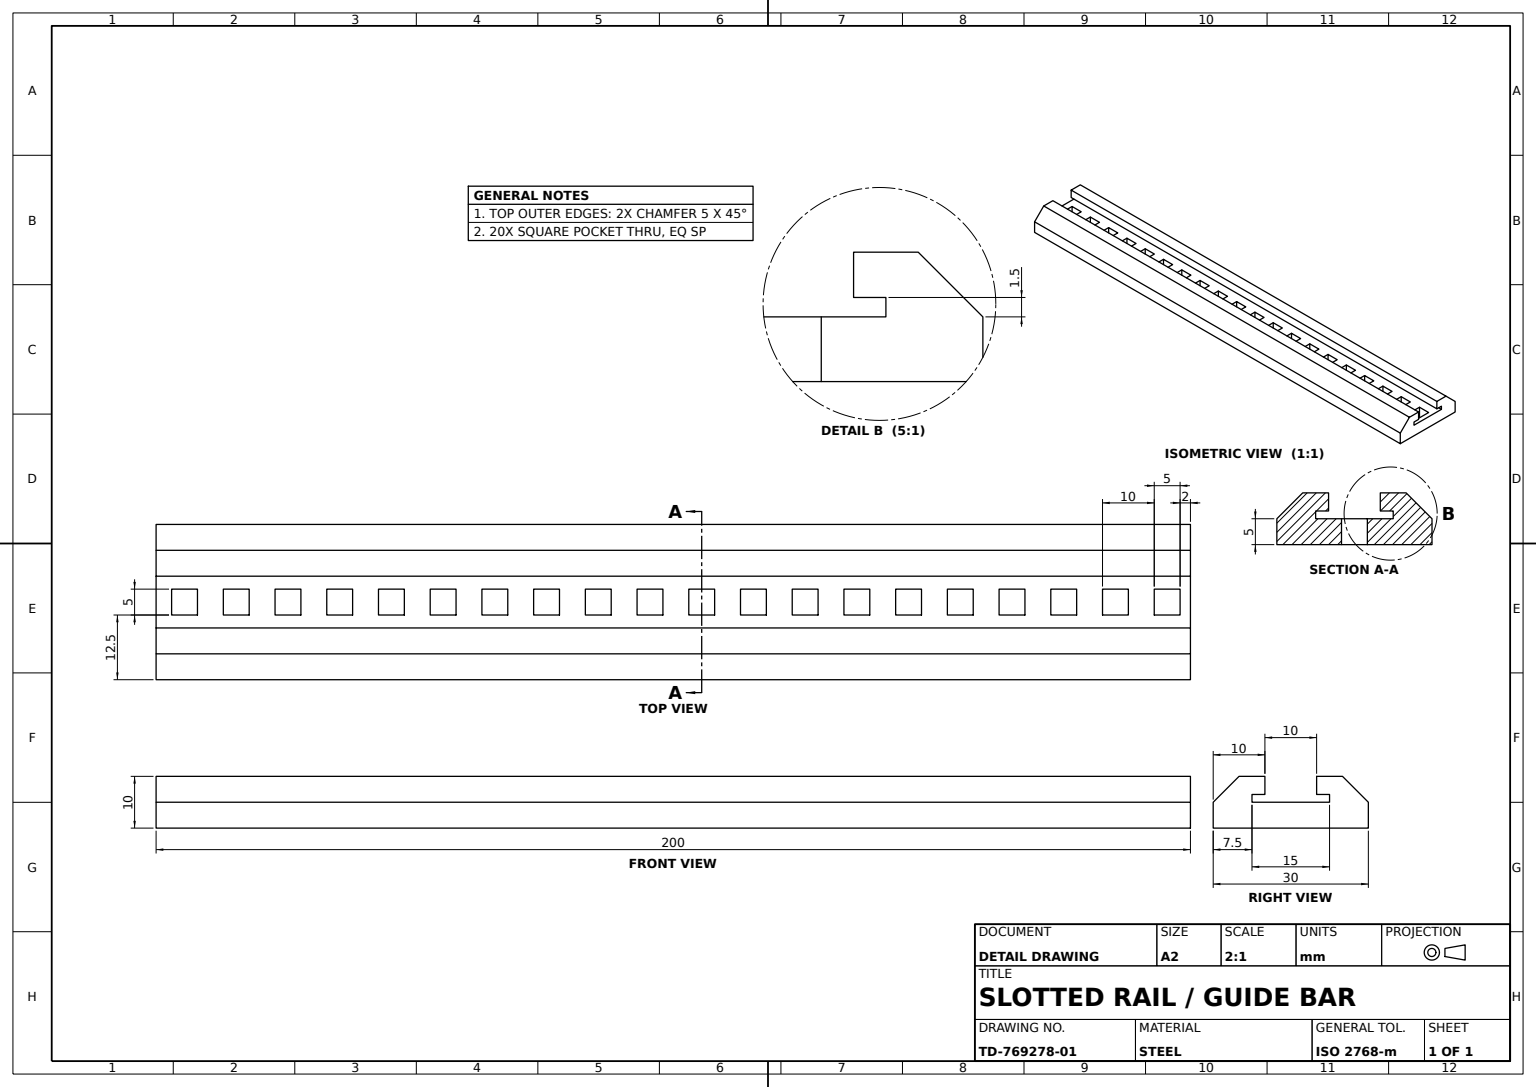
solid
v1 (2.5,-5,47)
v2 (2.5,0,47)
e1 v1 v2 LINE
v3 (2.5,0,42)
e2 v2 v3 LINE
v4 (2.5,-5,42)
e3 v4 v3 LINE
e4 v4 v1 LINE
face PLANE(AX(P(2.5,-5.001,42),D(1,0,0),D(0,0,-1))) rev [e1 e2 -e3 e4]
v5 (-2.5,-5,97)
v6 (-2.5,-5,92)
e5 v5 v6 LINE
v7 (-2.5,0,92)
e6 v6 v7 LINE
v8 (-2.5,0,97)
e7 v7 v8 LINE
e8 v5 v8 LINE
face PLANE(AX(P(-2.5,-5.001,92),D(-1,0,0),D(0,0,1))) rev [e5 e6 e7 -e8]
v9 (2.5,0,-48)
v10 (-2.5,0,-48)
e9 v9 v10 LINE
v11 (-2.5,-5,-48)
e10 v11 v10 LINE
v12 (2.5,-5,-48)
e11 v11 v12 LINE
e12 v12 v9 LINE
face PLANE(AX(P(-2.5,-5.001,-48),D(0,0,-1),D(-1,0,0))) rev [e9 -e10 e11 e12]
v13 (2.5,0,97)
v14 (2.5,0,92)
e13 v13 v14 LINE
v15 (2.5,-5,92)
e14 v15 v14 LINE
v16 (2.5,-5,97)
e15 v15 v16 LINE
e16 v16 v13 LINE
face PLANE(AX(P(2.5,-5.001,92),D(1,0,0),D(0,0,-1))) rev [e13 -e14 e15 e16]
v17 (-2.5,-5,32)
v18 (-2.5,0,32)
e17 v17 v18 LINE
v19 (2.5,-5,32)
e18 v17 v19 LINE
v20 (2.5,0,32)
e19 v19 v20 LINE
e20 v20 v18 LINE
face PLANE(AX(P(-2.5,-5.001,32),D(0,0,-1),D(-1,0,0))) rev [-e17 e18 e19 e20]
v21 (5,1.5,-100)
v22 (5,5,-100)
e21 v21 v22 LINE
v23 (5,1.5,100)
e22 v23 v21 LINE
v24 (5,5,100)
e23 v23 v24 LINE
e24 v24 v22 LINE
face PLANE(AX(P(5,0,-100),D(1,0,0),D(0,0,-1))) rev [-e21 -e22 e23 e24]
v25 (-2.5,-5,2)
v26 (-2.5,0,2)
e25 v25 v26 LINE
v27 (-2.5,0,7)
e26 v26 v27 LINE
v28 (-2.5,-5,7)
e27 v28 v27 LINE
e28 v28 v25 LINE
face PLANE(AX(P(-2.5,-5.001,2),D(-1,0,0),D(0,0,1))) rev [e25 e26 -e27 e28]
v29 (-5,1.5,100)
v30 (-7.5,1.5,100)
e29 v29 v30 LINE
v31 (-7.5,1.5,-100)
e30 v31 v30 LINE
v32 (-5,1.5,-100)
e31 v31 v32 LINE
e32 v32 v29 LINE
face PLANE(AX(P(-7.5,1.5,-100.001),D(0,1,0),D(0,0,1))) rev [e29 -e30 e31 e32]
v33 (-7.5,0,100)
e33 v30 v33 LINE
v34 (-7.5,0,-100)
e34 v34 v33 LINE
e35 v34 v31 LINE
face PLANE(AX(P(-7.5,1.5,-100.001),D(-1,0,0),D(0,0,1))) rev [e33 -e34 e35 e30]
v35 (-2.5,0,-33)
v36 (2.5,0,-33)
e36 v35 v36 LINE
v37 (2.5,-5,-33)
e37 v37 v36 LINE
v38 (-2.5,-5,-33)
e38 v37 v38 LINE
e39 v38 v35 LINE
face PLANE(AX(P(-2.5,-5.001,-33),D(0,0,1),D(1,0,0))) rev [e36 -e37 e38 e39]
v39 (-2.5,-5,-8)
v40 (-2.5,0,-8)
e40 v39 v40 LINE
v41 (-2.5,0,-3)
e41 v40 v41 LINE
v42 (-2.5,-5,-3)
e42 v42 v41 LINE
e43 v42 v39 LINE
face PLANE(AX(P(-2.5,-5.001,-8),D(-1,0,0),D(0,0,1))) rev [e40 e41 -e42 e43]
v43 (2.5,-5,-43)
e44 v12 v43 LINE
v44 (2.5,0,-43)
e45 v43 v44 LINE
e46 v44 v9 LINE
face PLANE(AX(P(2.5,-5.001,-48),D(1,0,0),D(0,0,-1))) rev [-e12 e44 e45 e46]
v45 (-2.5,-5,-28)
v46 (-2.5,0,-28)
e47 v45 v46 LINE
v47 (-2.5,0,-23)
e48 v46 v47 LINE
v48 (-2.5,-5,-23)
e49 v48 v47 LINE
e50 v48 v45 LINE
face PLANE(AX(P(-2.5,-5.001,-28),D(-1,0,0),D(0,0,1))) rev [e47 e48 -e49 e50]
v49 (-2.5,-5,87)
v50 (-2.5,0,87)
e51 v49 v50 LINE
v51 (-2.5,-5,82)
e52 v49 v51 LINE
v52 (-2.5,0,82)
e53 v51 v52 LINE
e54 v52 v50 LINE
face PLANE(AX(P(-2.5,-5.001,82),D(-1,0,0),D(0,0,1))) rev [-e51 e52 e53 e54]
v53 (-2.5,-5,-58)
v54 (-2.5,0,-58)
e55 v53 v54 LINE
v55 (-2.5,0,-53)
e56 v54 v55 LINE
v56 (-2.5,-5,-53)
e57 v56 v55 LINE
e58 v56 v53 LINE
face PLANE(AX(P(-2.5,-5.001,-58),D(-1,0,0),D(0,0,1))) rev [e55 e56 -e57 e58]
v57 (2.5,0,-83)
v58 (2.5,0,-88)
e59 v57 v58 LINE
v59 (2.5,-5,-88)
e60 v59 v58 LINE
v60 (2.5,-5,-83)
e61 v59 v60 LINE
e62 v60 v57 LINE
face PLANE(AX(P(2.5,-5.001,-88),D(1,0,0),D(0,0,-1))) rev [e59 -e60 e61 e62]
v61 (2.5,-5,2)
v62 (2.5,-5,7)
e63 v61 v62 LINE
v63 (2.5,0,7)
e64 v62 v63 LINE
v64 (2.5,0,2)
e65 v63 v64 LINE
e66 v61 v64 LINE
face PLANE(AX(P(2.5,-5.001,2),D(1,0,0),D(0,0,-1))) rev [e63 e64 e65 -e66]
v65 (-2.5,0,-43)
e67 v10 v65 LINE
v66 (-2.5,-5,-43)
e68 v66 v65 LINE
e69 v66 v11 LINE
face PLANE(AX(P(-2.5,-5.001,-48),D(-1,0,0),D(0,0,1))) rev [e10 e67 -e68 e69]
v67 (2.5,0,12)
v68 (-2.5,0,12)
e70 v67 v68 LINE
v69 (-2.5,-5,12)
e71 v69 v68 LINE
v70 (2.5,-5,12)
e72 v69 v70 LINE
e73 v70 v67 LINE
face PLANE(AX(P(-2.5,-5.001,12),D(0,0,-1),D(-1,0,0))) rev [e70 -e71 e72 e73]
v71 (2.5,0,67)
v72 (2.5,0,62)
e74 v71 v72 LINE
v73 (2.5,-5,62)
e75 v73 v72 LINE
v74 (2.5,-5,67)
e76 v73 v74 LINE
e77 v74 v71 LINE
face PLANE(AX(P(2.5,-5.001,62),D(1,0,0),D(0,0,-1))) rev [e74 -e75 e76 e77]
v75 (7.5,1.5,-100)
e78 v21 v75 LINE
v76 (7.5,1.5,100)
e79 v75 v76 LINE
e80 v76 v23 LINE
face PLANE(AX(P(-7.5,1.5,-100.001),D(0,1,0),D(0,0,1))) rev [e78 e79 e80 e22]
e81 v8 v13 LINE
e82 v16 v5 LINE
face PLANE(AX(P(-2.5,-5.001,97),D(0,0,1),D(1,0,0))) rev [e8 e81 -e16 e82]
v77 (2.5,0,-23)
v78 (2.5,0,-28)
e83 v77 v78 LINE
v79 (2.5,-5,-28)
e84 v79 v78 LINE
v80 (2.5,-5,-23)
e85 v79 v80 LINE
e86 v80 v77 LINE
face PLANE(AX(P(2.5,-5.001,-28),D(1,0,0),D(0,0,-1))) rev [e83 -e84 e85 e86]
v81 (-2.5,0,-68)
v82 (-2.5,0,-63)
e87 v81 v82 LINE
v83 (-2.5,-5,-63)
e88 v83 v82 LINE
v84 (-2.5,-5,-68)
e89 v83 v84 LINE
e90 v84 v81 LINE
face PLANE(AX(P(-2.5,-5.001,-68),D(-1,0,0),D(0,0,1))) rev [e87 -e88 e89 e90]
v85 (2.5,-5,22)
v86 (2.5,0,22)
e91 v85 v86 LINE
v87 (2.5,-5,27)
e92 v85 v87 LINE
v88 (2.5,0,27)
e93 v87 v88 LINE
e94 v88 v86 LINE
face PLANE(AX(P(2.5,-5.001,22),D(1,0,0),D(0,0,-1))) rev [-e91 e92 e93 e94]
v89 (2.5,-5,-93)
v90 (2.5,0,-93)
e95 v89 v90 LINE
v91 (2.5,0,-98)
e96 v90 v91 LINE
v92 (2.5,-5,-98)
e97 v92 v91 LINE
e98 v92 v89 LINE
face PLANE(AX(P(2.5,-5.001,-98),D(1,0,0),D(0,0,-1))) rev [e95 e96 -e97 e98]
v93 (2.5,-5,77)
v94 (-2.5,-5,77)
e99 v93 v94 LINE
v95 (-2.5,0,77)
e100 v94 v95 LINE
v96 (2.5,0,77)
e101 v95 v96 LINE
e102 v93 v96 LINE
face PLANE(AX(P(-2.5,-5.001,77),D(0,0,1),D(1,0,0))) rev [e99 e100 e101 -e102]
v97 (2.5,-5,-53)
v98 (2.5,0,-53)
e103 v97 v98 LINE
v99 (2.5,0,-58)
e104 v98 v99 LINE
v100 (2.5,-5,-58)
e105 v100 v99 LINE
e106 v100 v97 LINE
face PLANE(AX(P(2.5,-5.001,-58),D(1,0,0),D(0,0,-1))) rev [e103 e104 -e105 e106]
v101 (-2.5,0,37)
v102 (2.5,0,37)
e107 v101 v102 LINE
v103 (2.5,-5,37)
e108 v103 v102 LINE
v104 (-2.5,-5,37)
e109 v103 v104 LINE
e110 v104 v101 LINE
face PLANE(AX(P(-2.5,-5.001,37),D(0,0,1),D(1,0,0))) rev [e107 -e108 e109 e110]
v105 (-2.5,-5,-93)
v106 (-2.5,-5,-98)
e111 v105 v106 LINE
v107 (-2.5,0,-98)
e112 v106 v107 LINE
v108 (-2.5,0,-93)
e113 v107 v108 LINE
e114 v105 v108 LINE
face PLANE(AX(P(-2.5,-5.001,-98),D(-1,0,0),D(0,0,1))) rev [e111 e112 e113 -e114]
v109 (2.5,-5,52)
v110 (2.5,0,52)
e115 v109 v110 LINE
v111 (-2.5,0,52)
e116 v110 v111 LINE
v112 (-2.5,-5,52)
e117 v112 v111 LINE
e118 v112 v109 LINE
face PLANE(AX(P(-2.5,-5.001,52),D(0,0,-1),D(-1,0,0))) rev [e115 e116 -e117 e118]
e119 v62 v28 LINE
e120 v27 v63 LINE
face PLANE(AX(P(-2.5,-5.001,7),D(0,0,1),D(1,0,0))) rev [e119 e27 e120 -e64]
v113 (2.5,-5,-68)
v114 (2.5,0,-68)
e121 v113 v114 LINE
v115 (2.5,-5,-63)
e122 v113 v115 LINE
v116 (2.5,0,-63)
e123 v115 v116 LINE
e124 v116 v114 LINE
face PLANE(AX(P(2.5,-5.001,-68),D(1,0,0),D(0,0,-1))) rev [-e121 e122 e123 e124]
v117 (-2.5,-5,62)
v118 (-2.5,0,62)
e125 v117 v118 LINE
e126 v117 v73 LINE
e127 v72 v118 LINE
face PLANE(AX(P(-2.5,-5.001,62),D(0,0,-1),D(-1,0,0))) rev [-e125 e126 e75 e127]
v119 (15,0,-100)
v120 (15,0,100)
e128 v119 v120 LINE
v121 (10,5,-100)
e129 v121 v119 LINE
v122 (10,5,100)
e130 v122 v121 LINE
e131 v120 v122 LINE
face PLANE(AX(P(10,5,100),D(-0.707106781,-0.707106781,0),D(0,0,-1))) rev [-e128 -e129 -e130 -e131]
v123 (2.5,0,-38)
e132 v36 v123 LINE
v124 (2.5,-5,-38)
e133 v124 v123 LINE
e134 v124 v37 LINE
face PLANE(AX(P(2.5,-5.001,-38),D(1,0,0),D(0,0,-1))) rev [e132 -e133 e134 e37]
v125 (2.5,-5,-78)
v126 (2.5,-5,-73)
e135 v125 v126 LINE
v127 (2.5,0,-73)
e136 v126 v127 LINE
v128 (2.5,0,-78)
e137 v127 v128 LINE
e138 v125 v128 LINE
face PLANE(AX(P(2.5,-5.001,-78),D(1,0,0),D(0,0,-1))) rev [e135 e136 e137 -e138]
v129 (-5,5,-100)
v130 (-5,5,100)
e139 v129 v130 LINE
v131 (-10,5,-100)
e140 v129 v131 LINE
v132 (-10,5,100)
e141 v131 v132 LINE
e142 v130 v132 LINE
face PLANE(AX(P(-15,5,100),D(0,-1,0),D(0,0,-1))) rev [-e139 e140 e141 -e142]
v133 (2.5,-5,57)
v134 (-2.5,-5,57)
e143 v133 v134 LINE
v135 (-2.5,0,57)
e144 v134 v135 LINE
v136 (2.5,0,57)
e145 v135 v136 LINE
e146 v133 v136 LINE
face PLANE(AX(P(-2.5,-5.001,57),D(0,0,1),D(1,0,0))) rev [e143 e144 e145 -e146]
v137 (-2.5,-5,27)
v138 (-2.5,-5,22)
e147 v137 v138 LINE
v139 (-2.5,0,22)
e148 v138 v139 LINE
v140 (-2.5,0,27)
e149 v139 v140 LINE
e150 v137 v140 LINE
face PLANE(AX(P(-2.5,-5.001,22),D(-1,0,0),D(0,0,1))) rev [e147 e148 e149 -e150]
v141 (2.5,-5,-8)
v142 (2.5,-5,-3)
e151 v141 v142 LINE
v143 (2.5,0,-3)
e152 v142 v143 LINE
v144 (2.5,0,-8)
e153 v143 v144 LINE
e154 v141 v144 LINE
face PLANE(AX(P(2.5,-5.001,-8),D(1,0,0),D(0,0,-1))) rev [e151 e152 e153 -e154]
v145 (-2.5,-5,-83)
v146 (-2.5,0,-83)
e155 v145 v146 LINE
e156 v146 v57 LINE
e157 v60 v145 LINE
face PLANE(AX(P(-2.5,-5.001,-83),D(0,0,1),D(1,0,0))) rev [e155 e156 -e62 e157]
e158 v6 v15 LINE
e159 v14 v7 LINE
face PLANE(AX(P(-2.5,-5.001,92),D(0,0,-1),D(-1,0,0))) rev [-e6 e158 e14 e159]
e160 v104 v17 LINE
e161 v18 v101 LINE
face PLANE(AX(P(-2.5,-5.001,32),D(-1,0,0),D(0,0,1))) rev [e160 e17 e161 -e110]
v147 (7.5,0,100)
e162 v147 v76 LINE
v148 (7.5,0,-100)
e163 v75 v148 LINE
e164 v148 v147 LINE
face PLANE(AX(P(7.5,1.5,-100.001),D(1,0,0),D(0,0,-1))) rev [e162 -e79 e163 e164]
v149 (-2.5,-5,-38)
v150 (-2.5,0,-38)
e165 v149 v150 LINE
e166 v149 v124 LINE
e167 v123 v150 LINE
face PLANE(AX(P(-2.5,-5.001,-38),D(0,0,-1),D(-1,0,0))) rev [-e165 e166 e133 e167]
e168 v43 v66 LINE
e169 v65 v44 LINE
face PLANE(AX(P(-2.5,-5.001,-43),D(0,0,1),D(1,0,0))) rev [-e45 e168 e68 e169]
v151 (-2.5,-5,-73)
v152 (-2.5,0,-73)
e170 v151 v152 LINE
v153 (-2.5,-5,-78)
e171 v151 v153 LINE
v154 (-2.5,0,-78)
e172 v153 v154 LINE
e173 v154 v152 LINE
face PLANE(AX(P(-2.5,-5.001,-78),D(-1,0,0),D(0,0,1))) rev [-e170 e171 e172 e173]
e174 v111 v135 LINE
e175 v134 v112 LINE
face PLANE(AX(P(-2.5,-5.001,52),D(-1,0,0),D(0,0,1))) rev [e174 -e144 e175 e117]
e176 v114 v81 LINE
e177 v84 v113 LINE
face PLANE(AX(P(-2.5,-5.001,-68),D(0,0,-1),D(-1,0,0))) rev [e176 -e90 e177 e121]
e178 v38 v149 LINE
e179 v150 v35 LINE
face PLANE(AX(P(-2.5,-5.001,-38),D(-1,0,0),D(0,0,1))) rev [-e39 e178 e165 e179]
e180 v89 v105 LINE
e181 v108 v90 LINE
face PLANE(AX(P(-2.5,-5.001,-93),D(0,0,1),D(1,0,0))) rev [-e95 e180 e114 e181]
e182 v97 v56 LINE
e183 v55 v98 LINE
face PLANE(AX(P(-2.5,-5.001,-53),D(0,0,1),D(1,0,0))) rev [-e103 e182 e57 e183]
e184 v99 v54 LINE
e185 v53 v100 LINE
face PLANE(AX(P(-2.5,-5.001,-58),D(0,0,-1),D(-1,0,0))) rev [e184 -e55 e185 e105]
e186 v126 v151 LINE
e187 v153 v125 LINE
e188 v115 v83 LINE
v155 (2.5,-5,72)
e189 v155 v93 LINE
v156 (-2.5,-5,72)
e190 v156 v155 LINE
e191 v94 v156 LINE
v157 (-2.5,-5,17)
e192 v157 v69 LINE
v158 (2.5,-5,17)
e193 v158 v157 LINE
e194 v70 v158 LINE
e195 v25 v61 LINE
v159 (-2.5,-5,-18)
v160 (2.5,-5,-18)
e196 v159 v160 LINE
v161 (-2.5,-5,-13)
e197 v161 v159 LINE
v162 (2.5,-5,-13)
e198 v162 v161 LINE
e199 v160 v162 LINE
e200 v138 v85 LINE
e201 v87 v137 LINE
v163 (2.5,-5,82)
e202 v51 v163 LINE
v164 (2.5,-5,87)
e203 v164 v49 LINE
e204 v163 v164 LINE
v165 (-2.5,-5,67)
e205 v165 v117 LINE
e206 v74 v165 LINE
v166 (-15,-5,100)
v167 (15,-5,100)
e207 v166 v167 LINE
v168 (-15,-5,-100)
e208 v166 v168 LINE
v169 (15,-5,-100)
e209 v168 v169 LINE
e210 v167 v169 LINE
e211 v109 v133 LINE
e212 v45 v79 LINE
e213 v80 v48 LINE
v170 (-2.5,-5,42)
e214 v170 v4 LINE
v171 (-2.5,-5,47)
e215 v171 v170 LINE
e216 v1 v171 LINE
e217 v19 v103 LINE
e218 v106 v92 LINE
v172 (-2.5,-5,-88)
e219 v145 v172 LINE
e220 v172 v59 LINE
e221 v142 v42 LINE
e222 v39 v141 LINE
face PLANE(AX(P(-15,-5,100),D(0,1,0),D(0,0,1))) rev [-e171 -e186 -e135 -e187] [-e185 -e58 -e182 -e106] [-e188 -e122 -e177 -e89] [-e99 -e189 -e190 -e191] [-e72 -e192 -e193 -e194] [-e63 -e195 -e28 -e119] [-e196 -e197 -e198 -e199] [-e92 -e200 -e147 -e201] [-e11 -e69 -e168 -e44] [-e202 -e52 -e203 -e204] [-e126 -e205 -e206 -e76] [-e207 e208 e209 -e210] [-e143 -e211 -e118 -e175] [-e85 -e212 -e50 -e213] [-e4 -e214 -e215 -e216] [-e160 -e109 -e217 -e18] [-e98 -e218 -e111 -e180] [-e219 -e157 -e61 -e220] [-e221 -e151 -e222 -e43] [-e38 -e134 -e166 -e178] [-e15 -e158 -e5 -e82]
e223 v122 v24 LINE
e224 v121 v22 LINE
face PLANE(AX(P(-15,5,100),D(0,-1,0),D(0,0,-1))) rev [-e24 -e223 e130 e224]
v173 (2.5,0,72)
e225 v155 v173 LINE
e226 v96 v173 LINE
face PLANE(AX(P(2.5,-5.001,72),D(1,0,0),D(0,0,-1))) rev [-e225 e189 e102 e226]
v174 (-2.5,0,42)
e227 v3 v174 LINE
e228 v170 v174 LINE
face PLANE(AX(P(-2.5,-5.001,42),D(0,0,-1),D(-1,0,0))) rev [e214 e3 e227 -e228]
v175 (-2.5,0,-88)
e229 v172 v175 LINE
e230 v175 v146 LINE
face PLANE(AX(P(-2.5,-5.001,-88),D(-1,0,0),D(0,0,1))) rev [e219 e229 e230 -e155]
v176 (-2.5,0,67)
e231 v118 v176 LINE
e232 v165 v176 LINE
face PLANE(AX(P(-2.5,-5.001,62),D(-1,0,0),D(0,0,1))) rev [e125 e231 -e232 e205]
v177 (-2.5,0,-13)
v178 (2.5,0,-13)
e233 v177 v178 LINE
e234 v162 v178 LINE
e235 v161 v177 LINE
face PLANE(AX(P(-2.5,-5.001,-13),D(0,0,1),D(1,0,0))) rev [e233 -e234 e198 e235]
v179 (2.5,0,87)
e236 v164 v179 LINE
v180 (2.5,0,82)
e237 v179 v180 LINE
e238 v163 v180 LINE
face PLANE(AX(P(2.5,-5.001,82),D(1,0,0),D(0,0,-1))) rev [e204 e236 e237 -e238]
e239 v128 v154 LINE
face PLANE(AX(P(-2.5,-5.001,-78),D(0,0,-1),D(-1,0,0))) rev [-e172 e187 e138 e239]
e240 v180 v52 LINE
face PLANE(AX(P(-2.5,-5.001,82),D(0,0,-1),D(-1,0,0))) rev [e240 -e53 e202 e238]
e241 v169 v119 LINE
v181 (-15,0,-100)
e242 v181 v168 LINE
e243 v181 v131 LINE
e244 v32 v129 LINE
e245 v148 v34 LINE
face PLANE(AX(P(0,0,-100),D(0,0,1),D(1,0,0))) rev [-e224 e129 -e241 -e209 -e242 e243 -e140 -e244 -e31 -e35 -e245 -e163 -e78 e21]
e246 v144 v40 LINE
face PLANE(AX(P(-2.5,-5.001,-8),D(0,0,-1),D(-1,0,0))) rev [-e40 e222 e154 e246]
e247 v82 v116 LINE
face PLANE(AX(P(-2.5,-5.001,-63),D(0,0,1),D(1,0,0))) rev [e188 e88 e247 -e123]
e248 v167 v120 LINE
face PLANE(AX(P(15,5,100),D(-1,0,0),D(0,-1,0))) rev [e128 -e248 e210 e241]
e249 v64 v26 LINE
face PLANE(AX(P(-2.5,-5.001,2),D(0,0,-1),D(-1,0,0))) rev [e66 e249 -e25 e195]
e250 v50 v179 LINE
face PLANE(AX(P(-2.5,-5.001,87),D(0,0,1),D(1,0,0))) rev [e203 e51 e250 -e236]
v182 (-15,0,100)
e251 v132 v182 LINE
e252 v182 v166 LINE
e253 v33 v147 LINE
e254 v29 v130 LINE
face PLANE(AX(P(0,0,100),D(0,0,1),D(1,0,0))) [e251 e252 e207 e248 e131 e223 -e23 -e80 -e162 -e253 -e33 -e29 e254 e142]
e255 v58 v175 LINE
face PLANE(AX(P(-2.5,-5.001,-88),D(0,0,-1),D(-1,0,0))) rev [e220 e60 e255 -e229]
e256 v140 v88 LINE
face PLANE(AX(P(-2.5,-5.001,27),D(0,0,1),D(1,0,0))) rev [e201 e150 e256 -e93]
v183 (2.5,0,17)
e257 v158 v183 LINE
v184 (-2.5,0,17)
e258 v157 v184 LINE
e259 v184 v183 LINE
face PLANE(AX(P(-2.5,-5.001,17),D(0,0,1),D(1,0,0))) rev [-e257 e193 e258 e259]
e260 v68 v184 LINE
face PLANE(AX(P(-2.5,-5.001,12),D(-1,0,0),D(0,0,1))) rev [e192 e71 e260 -e258]
e261 v176 v71 LINE
face PLANE(AX(P(-2.5,-5.001,67),D(0,0,1),D(1,0,0))) rev [e232 e261 -e77 e206]
e262 v182 v181 LINE
face PLANE(AX(P(-15,0,100),D(0.707106781,-0.707106781,0),D(0,0,-1))) rev [-e243 -e262 -e251 -e141]
v185 (-2.5,0,47)
e263 v185 v2 LINE
e264 v171 v185 LINE
face PLANE(AX(P(-2.5,-5.001,47),D(0,0,1),D(1,0,0))) rev [e263 -e1 e216 e264]
e265 v47 v77 LINE
face PLANE(AX(P(-2.5,-5.001,-23),D(0,0,1),D(1,0,0))) rev [e213 e49 e265 -e86]
v186 (2.5,0,-18)
e266 v178 v186 LINE
e267 v160 v186 LINE
face PLANE(AX(P(2.5,-5.001,-18),D(1,0,0),D(0,0,-1))) rev [e266 -e267 e199 e234]
face PLANE(AX(P(-15,5,100),D(1,0,0),D(0,1,0))) rev [-e208 -e252 e262 e242]
e268 v152 v127 LINE
face PLANE(AX(P(-2.5,-5.001,-73),D(0,0,1),D(1,0,0))) rev [-e136 e186 e170 e268]
e269 v183 v67 LINE
face PLANE(AX(P(2.5,-5.001,12),D(1,0,0),D(0,0,-1))) rev [e194 e257 e269 -e73]
e270 v136 v110 LINE
face PLANE(AX(P(2.5,-5.001,52),D(1,0,0),D(0,0,-1))) rev [e146 e270 -e115 e211]
e271 v78 v46 LINE
face PLANE(AX(P(-2.5,-5.001,-28),D(0,0,-1),D(-1,0,0))) rev [-e47 e212 e84 e271]
e272 v41 v143 LINE
face PLANE(AX(P(-2.5,-5.001,-3),D(0,0,1),D(1,0,0))) rev [e42 e272 -e152 e221]
v187 (-2.5,0,-18)
e273 v159 v187 LINE
e274 v187 v177 LINE
face PLANE(AX(P(-2.5,-5.001,-18),D(-1,0,0),D(0,0,1))) rev [e197 e273 e274 -e235]
e275 v102 v20 LINE
face PLANE(AX(P(2.5,-5.001,32),D(1,0,0),D(0,0,-1))) rev [e217 e108 e275 -e19]
v188 (-2.5,0,72)
e276 v156 v188 LINE
e277 v188 v95 LINE
face PLANE(AX(P(-2.5,-5.001,72),D(-1,0,0),D(0,0,1))) rev [-e100 e191 e276 e277]
e278 v173 v188 LINE
face PLANE(AX(P(-2.5,-5.001,72),D(0,0,-1),D(-1,0,0))) rev [-e276 e190 e225 e278]
e279 v91 v107 LINE
face PLANE(AX(P(-2.5,-5.001,-98),D(0,0,-1),D(-1,0,0))) rev [-e112 e218 e97 e279]
e280 v174 v185 LINE
face PLANE(AX(P(-2.5,-5.001,42),D(-1,0,0),D(0,0,1))) rev [e280 -e264 e215 e228]
e281 v186 v187 LINE
e282 v86 v139 LINE
face PLANE(AX(P(0,0,0),D(0,1,0),D(0,0,1))) [-e161 -e20 -e275 -e107] [-e113 -e279 -e96 -e181] [-e127 -e74 -e261 -e231] [-e41 -e246 -e153 -e272] [-e281 -e266 -e233 -e274] [-e282 -e94 -e256 -e149] [-e124 -e247 -e87 -e176] [-e36 -e179 -e167 -e132] [-e277 -e278 -e226 -e101] [-e46 -e169 -e67 -e9] [-e230 -e255 -e59 -e156] [-e240 -e237 -e250 -e54] [-e227 -e2 -e263 -e280] [-e7 -e159 -e13 -e81] [-e48 -e271 -e83 -e265] [-e239 -e137 -e268 -e173] [-e174 -e116 -e270 -e145] [-e104 -e183 -e56 -e184] [-e120 -e26 -e249 -e65] [-e260 -e70 -e269 -e259] [e253 -e164 e245 e34]
face PLANE(AX(P(-2.5,-5.001,-18),D(0,0,-1),D(-1,0,0))) rev [e196 e267 e281 -e273]
face PLANE(AX(P(-5,0,-100),D(-1,0,0),D(0,0,1))) rev [-e254 -e32 e244 e139]
face PLANE(AX(P(-2.5,-5.001,22),D(0,0,-1),D(-1,0,0))) rev [e200 e91 e282 -e148]
